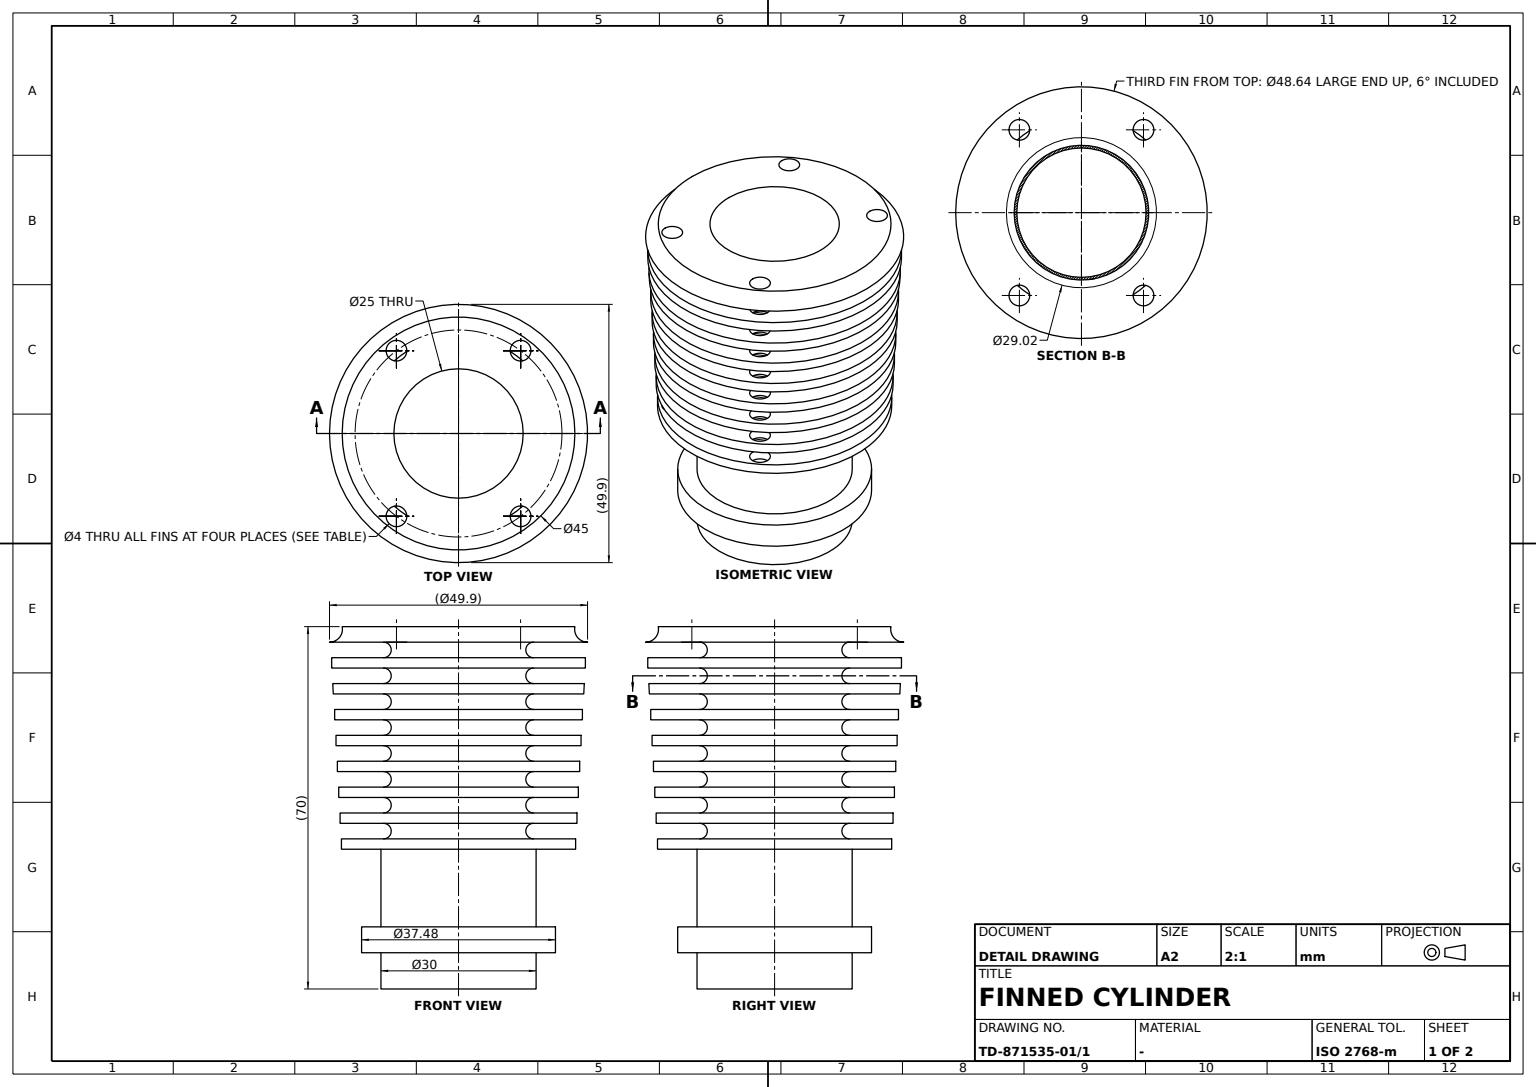
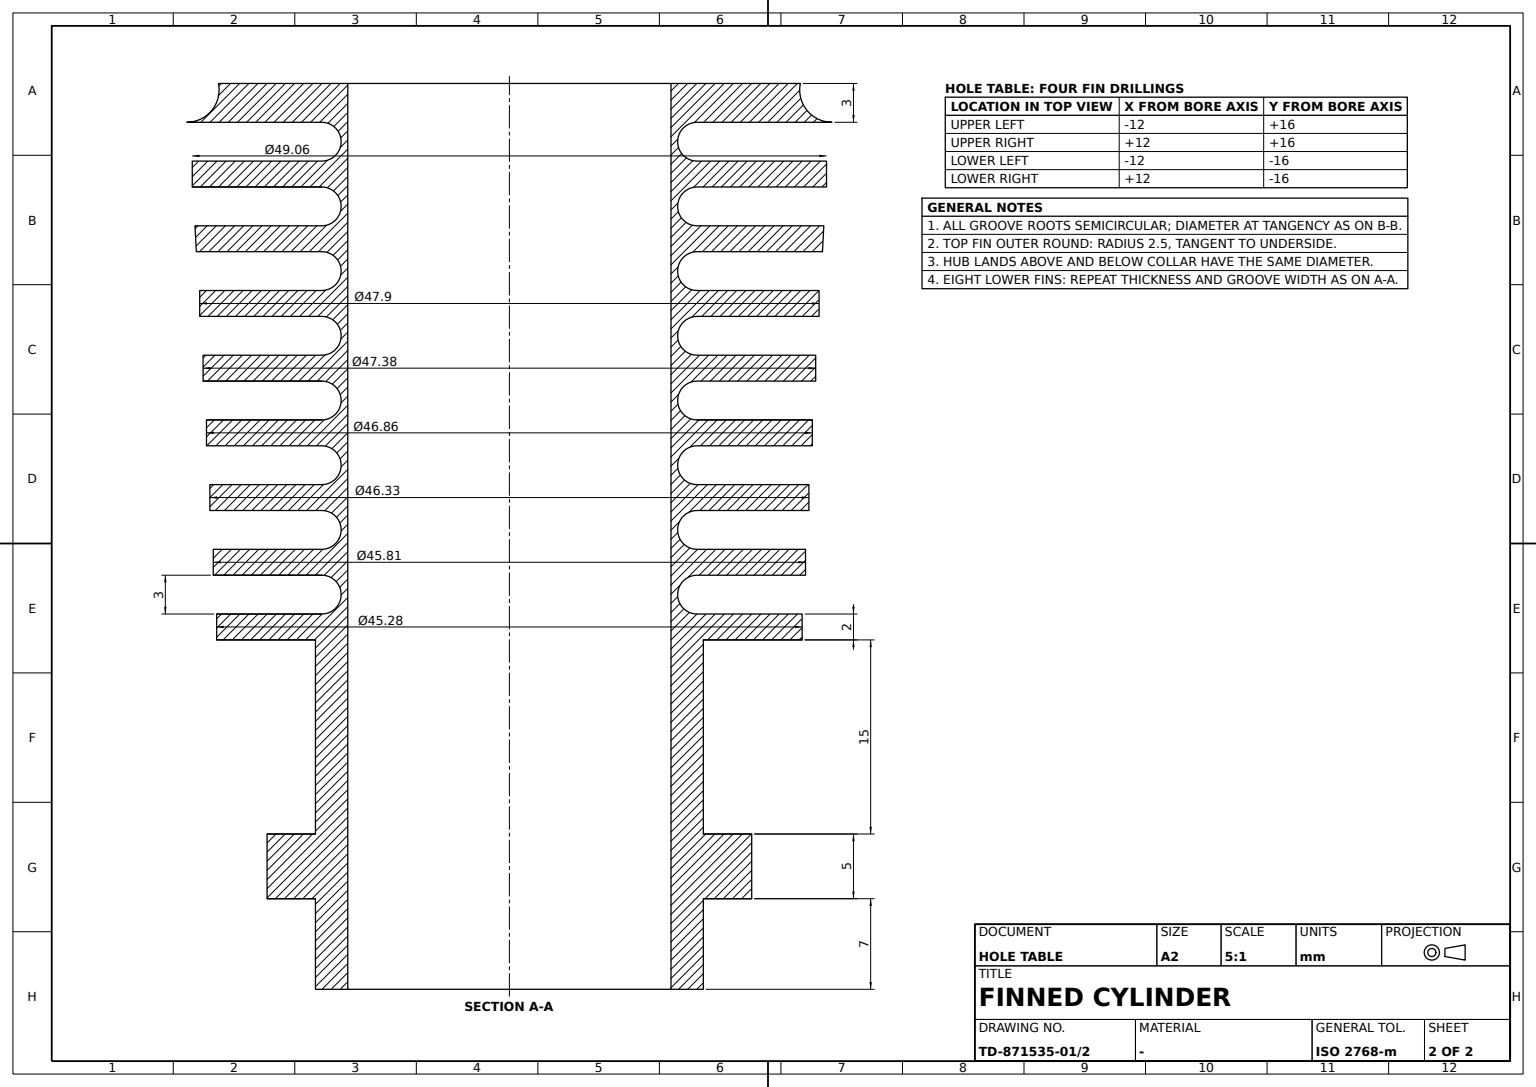
solid
v1 (-15,0,-35)
e1 v1 v1 CIRCLE(AX(P(0,0,-35),D(0,0,-1),D(-1,0,0)),15)
v2 (-12.5,0,-35)
e2 v2 v2 CIRCLE(AX(P(0,0,-35),D(0,0,-1),D(-1,0,0)),12.5)
face PLANE(AX(P(0,0,-35),D(0,0,-1),D(1,0,0))) [e1] [-e2]
v3 (10,-16,29)
e3 v3 v3 CIRCLE(AX(P(12,-16,29),D(0,0,-1),D(-1,0,0)),2)
v4 (10,-16,27)
e4 v4 v4 CIRCLE(AX(P(12,-16,27),D(0,0,-1),D(-1,0,0)),2)
face CYL(AX(P(12,-16,7.5),D(0,0,1),D(1,0,0)),2) rev [-e3] [e4]
v5 (-14,-16,4)
e5 v5 v5 CIRCLE(AX(P(-12,-16,4),D(0,0,-1),D(-1,0,0)),2)
v6 (-14,-16,2)
e6 v6 v6 CIRCLE(AX(P(-12,-16,2),D(0,0,-1),D(-1,0,0)),2)
face CYL(AX(P(-12,-16,7.5),D(0,0,1),D(1,0,0)),2) rev [-e5] [e6]
v7 (-14,-16,-3)
e7 v7 v7 CIRCLE(AX(P(-12,-16,-3),D(0,0,-1),D(-1,0,0)),2)
v8 (-14,-16,-1)
e8 v8 v8 CIRCLE(AX(P(-12,-16,-1),D(0,0,-1),D(-1,0,0)),2)
face CYL(AX(P(-12,-16,7.5),D(0,0,1),D(1,0,0)),2) rev [e7] [-e8]
v9 (-23.689806,0,14)
e9 v9 v9 CIRCLE(AX(P(0,0,14),D(0,0,-1),D(-1,0,0)),23.689806)
v10 (-23.689806,0,12)
e10 v10 v10 CIRCLE(AX(P(0,0,12),D(0,0,-1),D(-1,0,0)),23.689806)
face CYL(AX(P(0,0,0),D(0,0,-1),D(1,0,0)),23.689806) [e9] [-e10]
v11 (-14,16,-1)
e11 v11 v11 CIRCLE(AX(P(-12,16,-1),D(0,0,-1),D(-1,0,0)),2)
v12 (-14,16,-3)
e12 v12 v12 CIRCLE(AX(P(-12,16,-3),D(0,0,-1),D(-1,0,0)),2)
face CYL(AX(P(-12,16,7.5),D(0,0,1),D(1,0,0)),2) rev [-e11] [e12]
v13 (10,-16,-3)
e13 v13 v13 CIRCLE(AX(P(12,-16,-3),D(0,0,-1),D(-1,0,0)),2)
v14 (10,-16,-1)
e14 v14 v14 CIRCLE(AX(P(12,-16,-1),D(0,0,-1),D(-1,0,0)),2)
face CYL(AX(P(12,-16,7.5),D(0,0,1),D(1,0,0)),2) rev [e13] [-e14]
v15 (-14,-16,19)
e15 v15 v15 CIRCLE(AX(P(-12,-16,19),D(0,0,-1),D(-1,0,0)),2)
v16 (-14,-16,17)
e16 v16 v16 CIRCLE(AX(P(-12,-16,17),D(0,0,-1),D(-1,0,0)),2)
face CYL(AX(P(-12,-16,7.5),D(0,0,1),D(1,0,0)),2) rev [-e15] [e16]
v17 (10,16,22)
e17 v17 v17 CIRCLE(AX(P(12,16,22),D(0,0,-1),D(-1,0,0)),2)
v18 (10,16,24)
e18 v18 v18 CIRCLE(AX(P(12,16,24),D(0,0,-1),D(-1,0,0)),2)
face CYL(AX(P(12,16,7.5),D(0,0,1),D(1,0,0)),2) rev [e17] [-e18]
v19 (-14.512206,0,-3)
e19 v19 v19 CIRCLE(AX(P(0,0,-3),D(0,0,-1),D(-1,0,0)),14.512206)
v20 (-22.903689,0,-3)
e20 v20 v20 CIRCLE(AX(P(0,0,-3),D(0,0,-1),D(-1,0,0)),22.903689)
v21 (10,16,-3)
e21 v21 v21 CIRCLE(AX(P(12,16,-3),D(0,0,-1),D(-1,0,0)),2)
face PLANE(AX(P(-14.512206,0,-3),D(0,0,-1),D(1,0,0))) [-e12] [-e19] [e20] [-e21] [-e7] [-e13]
v22 (-14,16,17)
e22 v22 v22 CIRCLE(AX(P(-12,16,17),D(0,0,-1),D(-1,0,0)),2)
v23 (-23.951844,0,17)
e23 v23 v23 CIRCLE(AX(P(0,0,17),D(0,0,-1),D(-1,0,0)),23.951844)
v24 (-14.512206,0,17)
e24 v24 v24 CIRCLE(AX(P(0,0,17),D(0,0,-1),D(-1,0,0)),14.512206)
v25 (10,-16,17)
e25 v25 v25 CIRCLE(AX(P(12,-16,17),D(0,0,-1),D(-1,0,0)),2)
v26 (10,16,17)
e26 v26 v26 CIRCLE(AX(P(12,16,17),D(0,0,-1),D(-1,0,0)),2)
face PLANE(AX(P(-14.512206,0,17),D(0,0,-1),D(1,0,0))) [-e22] [e23] [-e24] [-e16] [-e25] [-e26]
v27 (-24.318699,0,24)
e27 v27 v27 CIRCLE(AX(P(0,0,24),D(0,0,-1),D(-1,0,0)),24.318699)
v28 (-24.213883,0,22)
e28 v28 v28 CIRCLE(AX(P(0,0,22),D(0,0,-1),D(-1,0,0)),24.213883)
face CONE(AX(P(0,0,22),D(0,0,1),D(1,0,0)),24.213883311,0.052359878) [e27] [-e28]
v29 (10,16,29)
e29 v29 v29 CIRCLE(AX(P(12,16,29),D(0,0,-1),D(-1,0,0)),2)
v30 (10,16,27)
e30 v30 v30 CIRCLE(AX(P(12,16,27),D(0,0,-1),D(-1,0,0)),2)
face CYL(AX(P(12,16,7.5),D(0,0,1),D(1,0,0)),2) rev [-e29] [e30]
v31 (-14,-16,22)
e31 v31 v31 CIRCLE(AX(P(-12,-16,22),D(0,0,-1),D(-1,0,0)),2)
v32 (-14,-16,24)
e32 v32 v32 CIRCLE(AX(P(-12,-16,24),D(0,0,-1),D(-1,0,0)),2)
face CYL(AX(P(-12,-16,7.5),D(0,0,1),D(1,0,0)),2) rev [e31] [-e32]
v33 (-22.903689,0,-1)
e33 v33 v33 CIRCLE(AX(P(0,0,-1),D(0,0,-1),D(-1,0,0)),22.903689)
v34 (10,16,-1)
e34 v34 v34 CIRCLE(AX(P(12,16,-1),D(0,0,-1),D(-1,0,0)),2)
v35 (-14.512206,0,-1)
e35 v35 v35 CIRCLE(AX(P(0,0,-1),D(0,0,-1),D(-1,0,0)),14.512206)
face PLANE(AX(P(-22.903689,0,-1),D(0,0,-1),D(1,0,0))) rev [-e33] [e14] [e8] [e34] [e11] [e35]
v36 (10,16,-6)
e36 v36 v36 CIRCLE(AX(P(12,16,-6),D(0,0,-1),D(-1,0,0)),2)
v37 (10,16,-8)
e37 v37 v37 CIRCLE(AX(P(12,16,-8),D(0,0,-1),D(-1,0,0)),2)
face CYL(AX(P(12,16,7.5),D(0,0,1),D(1,0,0)),2) rev [-e36] [e37]
v38 (-18.742436,0,-23)
e38 v38 v38 CIRCLE(AX(P(0,0,-23),D(0,0,-1),D(-1,0,0)),18.742436)
v39 (-18.742436,0,-28)
e39 v39 v39 CIRCLE(AX(P(0,0,-28),D(0,0,-1),D(-1,0,0)),18.742436)
face CYL(AX(P(0,0,0),D(0,0,-1),D(1,0,0)),18.742436) [e38] [-e39]
v40 (-14.512206,0,29)
e40 v40 v40 CIRCLE(AX(P(0,0,29),D(0,0,-1),D(-1,0,0)),14.512206)
v41 (-14.512206,0,32)
e41 v41 v41 CIRCLE(AX(P(0,0,32),D(0,0,-1),D(-1,0,0)),14.512206)
face TORUS(AX(P(0,0,30.5),D(0,0,-1),D(1,0,0)),14.512206,1.5) rev [-e40] [e41]
v42 (-14.512206,0,14)
e42 v42 v42 CIRCLE(AX(P(0,0,14),D(0,0,-1),D(-1,0,0)),14.512206)
face TORUS(AX(P(0,0,15.5),D(0,0,-1),D(1,0,0)),14.512206,1.5) rev [e24] [-e42]
v43 (10,16,32)
e43 v43 v43 CIRCLE(AX(P(12,16,32),D(0,0,-1),D(-1,0,0)),2)
v44 (10,16,35)
e44 v44 v44 CIRCLE(AX(P(12,16,35),D(0,0,-1),D(-1,0,0)),2) rev
face CYL(AX(P(12,16,7.5),D(0,0,1),D(1,0,0)),2) rev [e43] [e44]
v45 (10,-16,-6)
e45 v45 v45 CIRCLE(AX(P(12,-16,-6),D(0,0,-1),D(-1,0,0)),2)
v46 (-14,-16,-6)
e46 v46 v46 CIRCLE(AX(P(-12,-16,-6),D(0,0,-1),D(-1,0,0)),2)
v47 (-14,16,-6)
e47 v47 v47 CIRCLE(AX(P(-12,16,-6),D(0,0,-1),D(-1,0,0)),2)
v48 (-22.64165,0,-6)
e48 v48 v48 CIRCLE(AX(P(0,0,-6),D(0,0,-1),D(-1,0,0)),22.64165)
v49 (-14.512206,0,-6)
e49 v49 v49 CIRCLE(AX(P(0,0,-6),D(0,0,-1),D(-1,0,0)),14.512206)
face PLANE(AX(P(-22.64165,0,-6),D(0,0,-1),D(1,0,0))) rev [e45] [e46] [e36] [e47] [-e48] [e49]
face TORUS(AX(P(0,0,-4.5),D(0,0,-1),D(1,0,0)),14.512206,1.5) rev [-e49] [e19]
v50 (-14,-16,14)
e50 v50 v50 CIRCLE(AX(P(-12,-16,14),D(0,0,-1),D(-1,0,0)),2)
v51 (10,-16,14)
e51 v51 v51 CIRCLE(AX(P(12,-16,14),D(0,0,-1),D(-1,0,0)),2)
v52 (10,16,14)
e52 v52 v52 CIRCLE(AX(P(12,16,14),D(0,0,-1),D(-1,0,0)),2)
v53 (-14,16,14)
e53 v53 v53 CIRCLE(AX(P(-12,16,14),D(0,0,-1),D(-1,0,0)),2)
face PLANE(AX(P(-23.689806,0,14),D(0,0,-1),D(1,0,0))) rev [e42] [-e9] [e50] [e51] [e52] [e53]
v54 (-14,-16,9)
e54 v54 v54 CIRCLE(AX(P(-12,-16,9),D(0,0,-1),D(-1,0,0)),2)
v55 (-14,-16,7)
e55 v55 v55 CIRCLE(AX(P(-12,-16,7),D(0,0,-1),D(-1,0,0)),2)
face CYL(AX(P(-12,-16,7.5),D(0,0,1),D(1,0,0)),2) rev [-e54] [e55]
v56 (-14,16,32)
e56 v56 v56 CIRCLE(AX(P(-12,16,32),D(0,0,-1),D(-1,0,0)),2)
v57 (-14,16,35)
e57 v57 v57 CIRCLE(AX(P(-12,16,35),D(0,0,-1),D(-1,0,0)),2) rev
face CYL(AX(P(-12,16,7.5),D(0,0,1),D(1,0,0)),2) rev [e56] [e57]
v58 (-14,16,12)
e58 v58 v58 CIRCLE(AX(P(-12,16,12),D(0,0,-1),D(-1,0,0)),2)
v59 (-14.512206,0,12)
e59 v59 v59 CIRCLE(AX(P(0,0,12),D(0,0,-1),D(-1,0,0)),14.512206)
v60 (-14,-16,12)
e60 v60 v60 CIRCLE(AX(P(-12,-16,12),D(0,0,-1),D(-1,0,0)),2)
v61 (10,-16,12)
e61 v61 v61 CIRCLE(AX(P(12,-16,12),D(0,0,-1),D(-1,0,0)),2)
v62 (10,16,12)
e62 v62 v62 CIRCLE(AX(P(12,16,12),D(0,0,-1),D(-1,0,0)),2)
face PLANE(AX(P(-14.512206,0,12),D(0,0,-1),D(1,0,0))) [-e58] [e10] [-e59] [-e60] [-e61] [-e62]
v63 (-14,-16,32)
e63 v63 v63 CIRCLE(AX(P(-12,-16,32),D(0,0,-1),D(-1,0,0)),2)
v64 (10,-16,32)
e64 v64 v64 CIRCLE(AX(P(12,-16,32),D(0,0,-1),D(-1,0,0)),2)
v65 (-24.94949,0,32)
e65 v65 v65 CIRCLE(AX(P(0,0,32),D(0,0,-1),D(-1,0,0)),24.94949)
face PLANE(AX(P(-14.512206,0,32),D(0,0,-1),D(1,0,0))) [-e63] [-e56] [-e64] [-e41] [-e43] [e65]
v66 (-14.512206,0,24)
e66 v66 v66 CIRCLE(AX(P(0,0,24),D(0,0,-1),D(-1,0,0)),14.512206)
v67 (-14.512206,0,27)
e67 v67 v67 CIRCLE(AX(P(0,0,27),D(0,0,-1),D(-1,0,0)),14.512206)
face TORUS(AX(P(0,0,25.5),D(0,0,-1),D(1,0,0)),14.512206,1.5) rev [-e66] [e67]
v68 (10,-16,19)
e68 v68 v68 CIRCLE(AX(P(12,-16,19),D(0,0,-1),D(-1,0,0)),2)
v69 (-14,16,19)
e69 v69 v69 CIRCLE(AX(P(-12,16,19),D(0,0,-1),D(-1,0,0)),2)
v70 (-14.512206,0,19)
e70 v70 v70 CIRCLE(AX(P(0,0,19),D(0,0,-1),D(-1,0,0)),14.512206)
v71 (10,16,19)
e71 v71 v71 CIRCLE(AX(P(12,16,19),D(0,0,-1),D(-1,0,0)),2)
v72 (-23.951844,0,19)
e72 v72 v72 CIRCLE(AX(P(0,0,19),D(0,0,-1),D(-1,0,0)),23.951844)
face PLANE(AX(P(-23.951844,0,19),D(0,0,-1),D(1,0,0))) rev [e15] [e68] [e69] [e70] [e71] [-e72]
face CYL(AX(P(12,16,7.5),D(0,0,1),D(1,0,0)),2) rev [-e34] [e21]
v73 (-14,16,7)
e73 v73 v73 CIRCLE(AX(P(-12,16,7),D(0,0,-1),D(-1,0,0)),2)
v74 (-14,16,9)
e74 v74 v74 CIRCLE(AX(P(-12,16,9),D(0,0,-1),D(-1,0,0)),2)
face CYL(AX(P(-12,16,7.5),D(0,0,1),D(1,0,0)),2) rev [e73] [-e74]
v75 (-12.5,0,35)
e75 v75 v75 CIRCLE(AX(P(0,0,35),D(0,0,-1),D(-1,0,0)),12.5) rev
v76 (10,-16,35)
e76 v76 v76 CIRCLE(AX(P(12,-16,35),D(0,0,-1),D(-1,0,0)),2) rev
v77 (-22.5,0,35)
e77 v77 v77 CIRCLE(AX(P(0,0,35),D(0,0,-1),D(-1,0,0)),22.5)
v78 (-14,-16,35)
e78 v78 v78 CIRCLE(AX(P(-12,-16,35),D(0,0,-1),D(-1,0,0)),2) rev
face PLANE(AX(P(0,0,35),D(0,0,-1),D(1,0,0))) rev [-e44] [-e75] [-e57] [-e76] [-e77] [-e78]
v79 (-14.512206,0,22)
e79 v79 v79 CIRCLE(AX(P(0,0,22),D(0,0,-1),D(-1,0,0)),14.512206)
face TORUS(AX(P(0,0,20.5),D(0,0,-1),D(1,0,0)),14.512206,1.5) rev [e79] [-e70]
v80 (-14.512206,0,4)
e80 v80 v80 CIRCLE(AX(P(0,0,4),D(0,0,-1),D(-1,0,0)),14.512206)
v81 (-14.512206,0,7)
e81 v81 v81 CIRCLE(AX(P(0,0,7),D(0,0,-1),D(-1,0,0)),14.512206)
face TORUS(AX(P(0,0,5.5),D(0,0,-1),D(1,0,0)),14.512206,1.5) rev [-e80] [e81]
v82 (-14.512206,0,9)
e82 v82 v82 CIRCLE(AX(P(0,0,9),D(0,0,-1),D(-1,0,0)),14.512206)
face TORUS(AX(P(0,0,10.5),D(0,0,-1),D(1,0,0)),14.512206,1.5) rev [e59] [-e82]
v83 (-14,16,4)
e83 v83 v83 CIRCLE(AX(P(-12,16,4),D(0,0,-1),D(-1,0,0)),2)
v84 (-14,16,2)
e84 v84 v84 CIRCLE(AX(P(-12,16,2),D(0,0,-1),D(-1,0,0)),2)
face CYL(AX(P(-12,16,7.5),D(0,0,1),D(1,0,0)),2) rev [-e83] [e84]
face CYL(AX(P(12,16,7.5),D(0,0,1),D(1,0,0)),2) rev [e26] [-e71]
v85 (10,16,9)
e85 v85 v85 CIRCLE(AX(P(12,16,9),D(0,0,-1),D(-1,0,0)),2)
v86 (10,-16,9)
e86 v86 v86 CIRCLE(AX(P(12,-16,9),D(0,0,-1),D(-1,0,0)),2)
v87 (-23.427767,0,9)
e87 v87 v87 CIRCLE(AX(P(0,0,9),D(0,0,-1),D(-1,0,0)),23.427767)
face PLANE(AX(P(-23.427767,0,9),D(0,0,-1),D(1,0,0))) rev [e74] [e82] [e85] [e86] [-e87] [e54]
face CYL(AX(P(12,-16,7.5),D(0,0,1),D(1,0,0)),2) rev [e64] [e76]
face CYL(AX(P(0,0,7.5),D(0,0,1),D(1,0,0)),12.5) rev [e75] [e2]
v88 (-14,-16,27)
e88 v88 v88 CIRCLE(AX(P(-12,-16,27),D(0,0,-1),D(-1,0,0)),2)
v89 (-14,-16,29)
e89 v89 v89 CIRCLE(AX(P(-12,-16,29),D(0,0,-1),D(-1,0,0)),2)
face CYL(AX(P(-12,-16,7.5),D(0,0,1),D(1,0,0)),2) rev [e88] [-e89]
v90 (-15,0,-23)
e90 v90 v90 CIRCLE(AX(P(0,0,-23),D(0,0,-1),D(-1,0,0)),15)
face PLANE(AX(P(-18.742436,0,-23),D(0,0,-1),D(1,0,0))) rev [-e38] [e90]
v91 (10,16,7)
e91 v91 v91 CIRCLE(AX(P(12,16,7),D(0,0,-1),D(-1,0,0)),2)
v92 (10,-16,7)
e92 v92 v92 CIRCLE(AX(P(12,-16,7),D(0,0,-1),D(-1,0,0)),2)
v93 (-23.427767,0,7)
e93 v93 v93 CIRCLE(AX(P(0,0,7),D(0,0,-1),D(-1,0,0)),23.427767)
face PLANE(AX(P(-14.512206,0,7),D(0,0,-1),D(1,0,0))) [-e73] [-e91] [-e55] [-e92] [e93] [-e81]
face CYL(AX(P(12,-16,7.5),D(0,0,1),D(1,0,0)),2) rev [-e68] [e25]
v94 (10,-16,2)
e94 v94 v94 CIRCLE(AX(P(12,-16,2),D(0,0,-1),D(-1,0,0)),2)
v95 (10,-16,4)
e95 v95 v95 CIRCLE(AX(P(12,-16,4),D(0,0,-1),D(-1,0,0)),2)
face CYL(AX(P(12,-16,7.5),D(0,0,1),D(1,0,0)),2) rev [e94] [-e95]
face CYL(AX(P(12,-16,7.5),D(0,0,1),D(1,0,0)),2) rev [e61] [-e51]
face TORUS(AX(P(0,0,34.5),D(0,0,-1),D(1,0,0)),24.94949,2.5) rev [e77] [-e65]
face CYL(AX(P(12,-16,7.5),D(0,0,1),D(1,0,0)),2) rev [e92] [-e86]
face CYL(AX(P(-12,-16,7.5),D(0,0,1),D(1,0,0)),2) rev [-e50] [e60]
v96 (10,-16,24)
e96 v96 v96 CIRCLE(AX(P(12,-16,24),D(0,0,-1),D(-1,0,0)),2)
v97 (-14,16,24)
e97 v97 v97 CIRCLE(AX(P(-12,16,24),D(0,0,-1),D(-1,0,0)),2)
face PLANE(AX(P(-24.318699,0,24),D(0,0,-1),D(1,0,0))) rev [-e27] [e96] [e32] [e18] [e97] [e66]
v98 (10,-16,22)
e98 v98 v98 CIRCLE(AX(P(12,-16,22),D(0,0,-1),D(-1,0,0)),2)
face CYL(AX(P(12,-16,7.5),D(0,0,1),D(1,0,0)),2) rev [-e96] [e98]
face CYL(AX(P(-12,-16,7.5),D(0,0,1),D(1,0,0)),2) rev [e63] [e78]
v99 (-23.165728,0,2)
e99 v99 v99 CIRCLE(AX(P(0,0,2),D(0,0,-1),D(-1,0,0)),23.165728)
v100 (10,16,2)
e100 v100 v100 CIRCLE(AX(P(12,16,2),D(0,0,-1),D(-1,0,0)),2)
v101 (-14.512206,0,2)
e101 v101 v101 CIRCLE(AX(P(0,0,2),D(0,0,-1),D(-1,0,0)),14.512206)
face PLANE(AX(P(-14.512206,0,2),D(0,0,-1),D(1,0,0))) [-e94] [e99] [-e84] [-e6] [-e100] [-e101]
face CYL(AX(P(12,16,7.5),D(0,0,1),D(1,0,0)),2) rev [e62] [-e52]
v102 (-23.165728,0,4)
e102 v102 v102 CIRCLE(AX(P(0,0,4),D(0,0,-1),D(-1,0,0)),23.165728)
v103 (10,16,4)
e103 v103 v103 CIRCLE(AX(P(12,16,4),D(0,0,-1),D(-1,0,0)),2)
face PLANE(AX(P(-23.165728,0,4),D(0,0,-1),D(1,0,0))) rev [-e102] [e5] [e103] [e83] [e80] [e95]
face CYL(AX(P(12,16,7.5),D(0,0,1),D(1,0,0)),2) rev [-e85] [e91]
v104 (-14,16,29)
e104 v104 v104 CIRCLE(AX(P(-12,16,29),D(0,0,-1),D(-1,0,0)),2)
v105 (-24.527748,0,29)
e105 v105 v105 CIRCLE(AX(P(0,0,29),D(0,0,-1),D(-1,0,0)),24.527748)
face PLANE(AX(P(-24.527748,0,29),D(0,0,-1),D(1,0,0))) rev [e104] [e89] [e40] [e29] [-e105] [e3]
v106 (-14,16,27)
e106 v106 v106 CIRCLE(AX(P(-12,16,27),D(0,0,-1),D(-1,0,0)),2)
face CYL(AX(P(-12,16,7.5),D(0,0,1),D(1,0,0)),2) rev [e106] [-e104]
face TORUS(AX(P(0,0,0.5),D(0,0,-1),D(1,0,0)),14.512206,1.5) rev [e101] [-e35]
v107 (-15,0,-8)
e107 v107 v107 CIRCLE(AX(P(0,0,-8),D(0,0,-1),D(-1,0,0)),15)
v108 (10,-16,-8)
e108 v108 v108 CIRCLE(AX(P(12,-16,-8),D(0,0,-1),D(-1,0,0)),2)
v109 (-14,16,-8)
e109 v109 v109 CIRCLE(AX(P(-12,16,-8),D(0,0,-1),D(-1,0,0)),2)
v110 (-22.64165,0,-8)
e110 v110 v110 CIRCLE(AX(P(0,0,-8),D(0,0,-1),D(-1,0,0)),22.64165)
v111 (-14,-16,-8)
e111 v111 v111 CIRCLE(AX(P(-12,-16,-8),D(0,0,-1),D(-1,0,0)),2)
face PLANE(AX(P(-15,0,-8),D(0,0,-1),D(1,0,0))) [-e107] [-e37] [-e108] [-e109] [e110] [-e111]
v112 (-24.527748,0,27)
e112 v112 v112 CIRCLE(AX(P(0,0,27),D(0,0,-1),D(-1,0,0)),24.527748)
face CYL(AX(P(0,0,0),D(0,0,-1),D(1,0,0)),24.527748) [e105] [-e112]
face CYL(AX(P(12,16,7.5),D(0,0,1),D(1,0,0)),2) rev [e100] [-e103]
v113 (-15,0,-28)
e113 v113 v113 CIRCLE(AX(P(0,0,-28),D(0,0,-1),D(-1,0,0)),15)
face CYL(AX(P(0,0,0),D(0,0,-1),D(1,0,0)),15) [e113] [-e1]
v114 (-14,16,22)
e114 v114 v114 CIRCLE(AX(P(-12,16,22),D(0,0,-1),D(-1,0,0)),2)
face CYL(AX(P(-12,16,7.5),D(0,0,1),D(1,0,0)),2) rev [e114] [-e97]
face CYL(AX(P(0,0,0),D(0,0,-1),D(1,0,0)),23.951844) [e72] [-e23]
face CYL(AX(P(-12,16,7.5),D(0,0,1),D(1,0,0)),2) rev [e58] [-e53]
face CYL(AX(P(0,0,0),D(0,0,-1),D(1,0,0)),23.427767) [e87] [-e93]
face CYL(AX(P(-12,16,7.5),D(0,0,1),D(1,0,0)),2) rev [-e69] [e22]
face CYL(AX(P(-12,16,7.5),D(0,0,1),D(1,0,0)),2) rev [e109] [-e47]
face CYL(AX(P(0,0,0),D(0,0,-1),D(1,0,0)),15) [-e90] [e107]
face PLANE(AX(P(-14.512206,0,22),D(0,0,-1),D(1,0,0))) [-e17] [-e114] [-e98] [-e79] [-e31] [e28]
face PLANE(AX(P(-14.512206,0,27),D(0,0,-1),D(1,0,0))) [-e88] [-e67] [-e106] [e112] [-e4] [-e30]
face CYL(AX(P(0,0,0),D(0,0,-1),D(1,0,0)),23.165728) [-e99] [e102]
face CYL(AX(P(-12,-16,7.5),D(0,0,1),D(1,0,0)),2) rev [-e46] [e111]
face CYL(AX(P(0,0,0),D(0,0,-1),D(1,0,0)),22.903689) [-e20] [e33]
face CYL(AX(P(0,0,0),D(0,0,-1),D(1,0,0)),22.64165) [-e110] [e48]
face PLANE(AX(P(-15,0,-28),D(0,0,-1),D(1,0,0))) [-e113] [e39]
face CYL(AX(P(12,-16,7.5),D(0,0,1),D(1,0,0)),2) rev [e108] [-e45]
